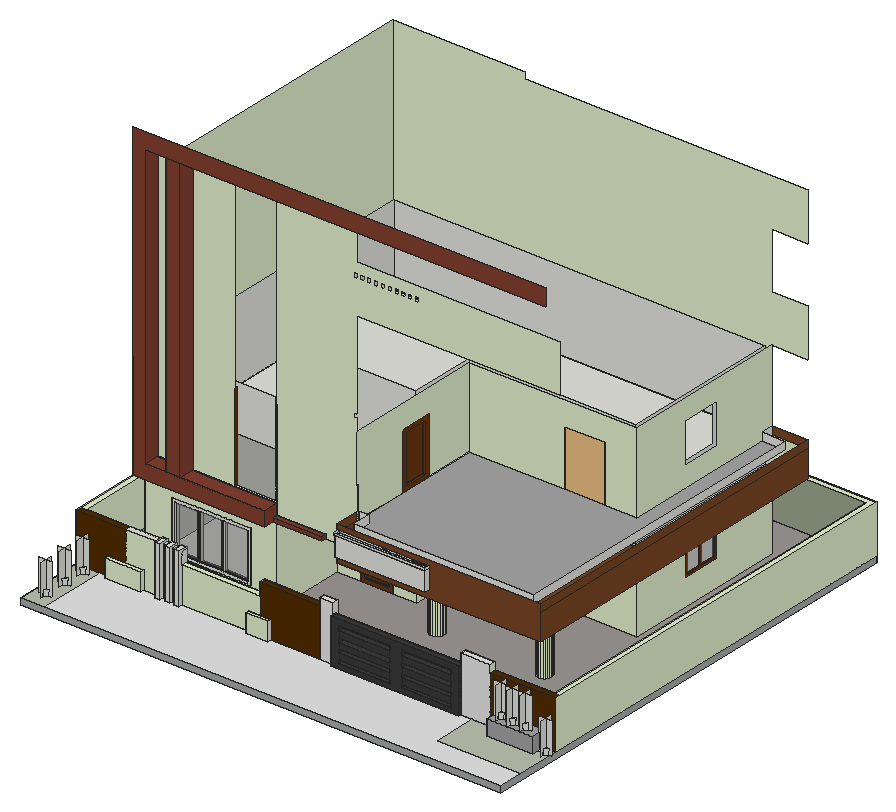
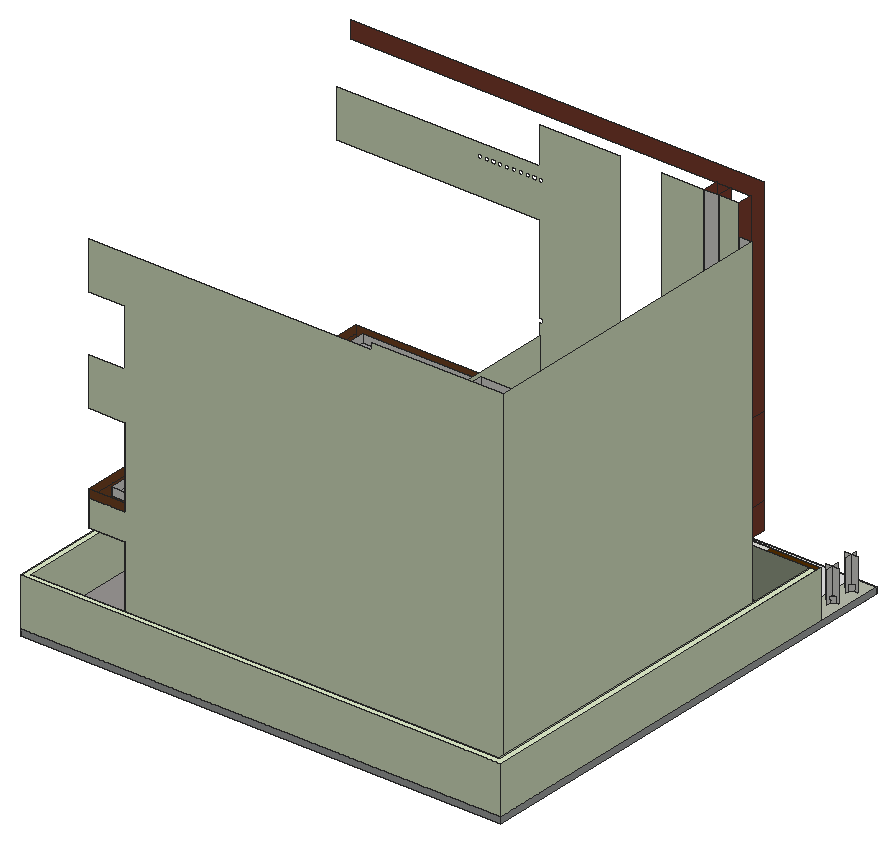
# SketchUp Ruby script. Lengths in inches.
U = 1.inch
M = Sketchup.active_model
def pt(a) = Geom::Point3d.new(a.map { |v| v * U })
def face(e, loops, mat)
  f = e.add_face(loops[0].map { |a| pt(a) })
  loops[1..].each { |l| e.add_face(l.map { |a| pt(a) }).erase! }
  f.material = f.back_material = mat if mat
  f
end
# faces: each face lists its corners as indices into pts; further lists are holes
def faces(e, pts, list, mat = nil) = list.each { |f| face(e, (f[0].is_a?(Array) ? f : [f]).map { |l| l.map { |i| pts[i] } }, mat) }
# xy, xz, yz: faces in a plane at the given z, y or x. An outline is a flat list of corners, or four numbers for a rectangle; further outlines are holes
def ring(l) = l.size == 4 ? [[l[0], l[1]], [l[2], l[1]], [l[2], l[3]], [l[0], l[3]]] : l.each_slice(2).to_a
def flat(e, list, mat, &to3) = list.each { |f| face(e, (f[0].is_a?(Array) ? f : [f]).map { |l| ring(l).map { |u, v| to3.(u, v) } }, mat) }
def xy(e, z, list, mat = nil) = flat(e, list, mat) { |x, y| [x, y, z] }
def xz(e, y, list, mat = nil) = flat(e, list, mat) { |x, z| [x, y, z] }
def yz(e, x, list, mat = nil) = flat(e, list, mat) { |y, z| [x, y, z] }
def lines(e, pts, list) = list.each { |a, b| e.add_line(pt(pts[a]), pt(pts[b])) }
# prism: a flat outline (further loops are holes) pulled along v
def prism(e, loops, v, mat = nil)
  f = face(e, loops, mat); d = Geom::Vector3d.new(v.map { |x| x * U })
  f.pushpull(f.normal.samedirection?(d) ? d.length : -d.length)
end
def box(e, o, s, mat = nil) = prism(e, [[o, [o[0] + s[0], o[1], o[2]], [o[0] + s[0], o[1] + s[1], o[2]], [o[0], o[1] + s[1], o[2]]]], [0, 0, s[2]], mat)
def at(x, y, z, deg = 0) = Geom::Transformation.translation(pt([x, y, z])) * Geom::Transformation.rotation(ORIGIN, Z_AXIS, deg.degrees)
def axes(o, x, y, z) = Geom::Transformation.new([*x, 0, *y, 0, *z, 0, *pt(o).to_a, 1])
def part(name) = M.definitions.add(name)
# library, detail: a bought-in or finely detailed component or shape, given as its bounding box
def library(name, o, s) = part(name).tap { |d| box(d.entities, o, s) }
def detail(e, o, s) = box(e.add_group.entities, o, s)
def put(e, d, t, mat = nil) = e.add_instance(d, t).tap { |i| i.material = mat if mat }
def group(e, t, mat = nil) = e.add_group.tap { |g| g.transformation = t; g.material = mat if mat }.entities
root = M.entities
M.materials.add("[Color A08]").color = [102, 52, 0]
M.materials.add("[Color C08]").color = [82, 45, 0]
M.materials.add("[Color M00]").color = [255, 255, 255]
M.materials.add("[Color M07]").color = [58, 58, 58]
M.materials.add("[Concrete Aggregate Smoke]").color = [154, 150, 148]
M.materials.add("[Concrete Form 4x8]").color = [167, 170, 168]
M.materials.add("[Mirror 01]").color = [185, 185, 181]
M.materials.add("[Pavers Flagstone Gray]").color = [162, 162, 162]
M.materials.add("[Pavers with Grass Brick]").color = [187, 192, 176]
M.materials.add("[Polished Concrete Old]").color = [229, 229, 229]
M.materials.add("[Stone Vein Gray]").color = [166, 165, 165]
M.materials.add("[Translucent Glass Gray]").color = [128, 128, 128]
M.materials["[Translucent Glass Gray]"].alpha = 0.5
M.materials.add("[Wood Board Cork]").color = [130, 63, 47]
M.materials.add("[Wood Lumber ButtJoined]").color = [225, 238, 204]
M.materials.add("[Wood Lumber ButtJoined]1").color = [154, 164, 141]
M.materials.add("[Wood Veneer 01]1").color = [120, 70, 37]
M.materials.add("[Wood Veneer 02]").color = [107, 55, 17]
c1 = part("Gruppe\#59")
xz(c1.entities,0,[[0,0,19.69,47.24]])
c2 = part("Gruppe\#58")
xz(c2.entities,0,[[0,0,19.69,47.24]])
c3 = part("buchsbaum")
xy(c3.entities,8.86,[[9.1875,3.27,15.1,9.1875,9.1875,15.1,3.27,9.1875]])
p = [[9.1875,4.45,0],[9.1875,3.27,8.86],[3.27,9.1875,8.86],[4.45,9.1875,0],[13.92,9.1875,0],[15.1,9.1875,8.86],
  [9.1875,15.1,8.86],[9.1875,13.92,0]]
faces(c3.entities,p,[[0,1,2,3],[4,5,1,0],[3,2,6,7],[7,6,5,4]])
put(c3.entities,c1,at(0,9.84,0))
put(c3.entities,c2,at(9.84,0,0,90))
c4 = part("Group\#3")
xy(c4.entities,0,[[0,0,48,3.1875]],"[Wood Veneer 02]")
xy(c4.entities,5.53,[[5.53,0,42.47,3.1875]],"[Wood Veneer 02]")
xy(c4.entities,78.47,[[5.53,0,42.47,3.1875]],"[Wood Veneer 02]")
xy(c4.entities,84,[[0,0,48,3.1875]],"[Wood Veneer 02]")
xz(c4.entities,0,[[[0,0,48,84],[5.53,5.53,42.47,78.47]]],"[Wood Veneer 02]")
xz(c4.entities,3.1875,[[[0,0,48,84],[5.53,5.53,42.47,78.47]],[5.53,5.53,42.47,78.47]],"[Wood Veneer 02]")
yz(c4.entities,0,[[0,0,3.1875,84]],"[Wood Veneer 02]")
yz(c4.entities,5.53,[[0,5.53,3.1875,78.47]],"[Wood Veneer 02]")
yz(c4.entities,42.47,[[0,5.53,3.1875,78.47]],"[Wood Veneer 02]")
yz(c4.entities,48,[[0,0,3.1875,84]],"[Wood Veneer 02]")
c5 = part("Group\#4")
xy(c5.entities,0,[[0,0,21.9375,1.125]],"[Wood Veneer 02]")
xy(c5.entities,1.52,[[1.52,0,10.45,1.125],[10.97,0,20.42,1.125]],"[Wood Veneer 02]")
xy(c5.entities,22.11,[[1.52,0,10.45,1.125],[10.97,0,20.42,1.125]],"[Wood Veneer 02]")
xy(c5.entities,23.625,[[0,0,21.9375,1.125]],"[Wood Veneer 02]")
xz(c5.entities,0,[[[0,0,21.9375,23.625],[10.97,1.52,20.42,22.11],[1.52,1.52,10.45,22.11]]],"[Wood Veneer 02]")
xz(c5.entities,1.125,[[1.52,1.52,10.45,22.11],[10.97,1.52,20.42,22.11]],"[Translucent Glass Gray]")
xz(c5.entities,1.125,[[[0,0,21.9375,23.625],[10.97,1.52,20.42,22.11],[1.52,1.52,10.45,22.11]]],"[Wood Veneer 02]")
yz(c5.entities,0,[[0,0,1.125,23.625]],"[Wood Veneer 02]")
yz(c5.entities,1.52,[[0,1.52,1.125,22.11]],"[Wood Veneer 02]")
yz(c5.entities,10.45,[[0,1.52,1.125,22.11]],"[Wood Veneer 02]")
yz(c5.entities,10.97,[[0,1.52,1.125,22.11]],"[Wood Veneer 02]")
yz(c5.entities,20.42,[[0,1.52,1.125,22.11]],"[Wood Veneer 02]")
yz(c5.entities,21.9375,[[0,0,1.125,23.625]],"[Wood Veneer 02]")
c6 = part("Group\#2")
xy(c6.entities,0,[[0,0,48,3.1875]],"[Wood Veneer 02]")
xy(c6.entities,5.53,[[5.53,0,42.47,3.1875]],"[Wood Veneer 02]")
xy(c6.entities,78.47,[[5.53,0,42.47,3.1875]],"[Wood Veneer 02]")
xy(c6.entities,84,[[0,0,48,3.1875]],"[Wood Veneer 02]")
xz(c6.entities,0,[[[0,0,48,84],[5.53,5.53,42.47,78.47]]],"[Wood Veneer 02]")
xz(c6.entities,3.1875,[[[0,0,48,84],[5.53,5.53,42.47,78.47]],[5.53,5.53,42.47,78.47]],"[Wood Veneer 02]")
yz(c6.entities,0,[[0,0,3.1875,84]],"[Wood Veneer 02]")
yz(c6.entities,5.53,[[0,5.53,3.1875,78.47]],"[Wood Veneer 02]")
yz(c6.entities,42.47,[[0,5.53,3.1875,78.47]],"[Wood Veneer 02]")
yz(c6.entities,48,[[0,0,3.1875,84]],"[Wood Veneer 02]")
c7 = library("Group\#5",[0,0,0],[60,3.4375,84])
xy(root,0,[[0,0,720,704.375]],"[Concrete Form 4x8]")
xy(root,9,[[47.625,99.125,47.625,104.375,0,104.375,0,704.375,720,704.375,720,104.375,576.98,104.375,576.98,113.375,711,113.375,711,695.375,9,695.375,9,113.375,365.09,113.375,365.09,104.375,101.5,104.375,101.5,99.125],[122.78,99.125,130.4,104.375],[136.78,99.125,144.4,104.375],[150.84,99.125,158.46,104.375],[258.67,99.125,291.92,104.375],
  [53.1875,166.9375,53.1875,631.8125,621.4375,631.8125,621.4375,378.5,543.9375,378.5,543.9375,384.5,615.4375,384.5,615.4375,625.8125,59.1875,625.8125,59.1875,172.9375,245.25,172.9375,245.25,286.0625,286.51,286.0625,286.51,280.0625,251.25,280.0625,251.25,166.9375],[59.1875,172.9375,245.25,172.9375,245.25,286.0625,364.4375,286.0625,364.4375,384.5,615.4375,384.5,615.4375,625.8125,59.1875,625.8125],[431.7,230.58,428.91,230.95,426.32,232.03,424.09,233.73,422.39,235.96,421.3125,238.55,420.95,241.33,421.3125,244.12,422.39,246.71,424.09,248.9375,426.32,250.64,428.91,251.72,431.7,252.08,434.48,251.72,437.07,250.64,439.3,248.9375,441.01,246.71,442.08,244.12,442.45,241.33,442.08,238.55,441.01,235.96,439.3,233.73,437.07,232.03,434.48,230.95],[593.38,230.58,590.6,230.95,588.01,232.03,585.78,233.73,584.07,235.96,583,238.55,582.63,241.33,583,244.12,584.07,246.71,585.78,248.9375,588.01,250.64,590.6,251.72,593.38,252.08,596.17,251.72,598.76,250.64,600.98,248.9375,602.69,246.71,603.77,244.12,604.13,241.33,603.77,238.55,602.69,235.96,600.98,233.73,598.76,232.03,596.17,230.95],[334.51,280.0625,334.51,286.0625,364.4375,286.0625,364.4375,311.76,370.4375,311.76,370.4375,280.0625],
  [364.4375,347.76,364.4375,384.5,495.9375,384.5,495.9375,378.5,370.4375,378.5,370.4375,347.76]])
xy(root,9,[[365.09,104.375,385.78,113.375]],"[Color M00]")
xy(root,9,[[[9,113.375,711,695.375],[53.1875,166.9375,53.1875,631.8125,621.4375,631.8125,621.4375,378.5,543.9375,378.5,543.9375,384.5,495.9375,384.5,495.9375,378.5,370.4375,378.5,370.4375,347.76,364.4375,347.76,364.4375,311.76,370.4375,311.76,370.4375,280.0625,334.51,280.0625,334.51,286.0625,286.51,286.0625,286.51,280.0625,251.25,280.0625,251.25,166.9375],[431.7,230.58,428.91,230.95,426.32,232.03,424.09,233.73,422.39,235.96,421.3125,238.55,420.95,241.33,421.3125,244.12,422.39,246.71,424.09,248.9375,426.32,250.64,428.91,251.72,431.7,252.08,434.48,251.72,437.07,250.64,439.3,248.9375,441.01,246.71,442.08,244.12,442.45,241.33,442.08,238.55,441.01,235.96,439.3,233.73,437.07,232.03,434.48,230.95],[593.38,230.58,590.6,230.95,588.01,232.03,585.78,233.73,584.07,235.96,583,238.55,582.63,241.33,583,244.12,584.07,246.71,585.78,248.9375,588.01,250.64,590.6,251.72,593.38,252.08,596.17,251.72,598.76,250.64,600.98,248.9375,602.69,246.71,603.77,244.12,604.13,241.33,603.77,238.55,602.69,235.96,600.98,233.73,598.76,232.03,596.17,230.95]]],"[Concrete Aggregate Smoke]")
xy(root,9,[[633.14,82.625,701.76,104.375]],"[Pavers Flagstone Gray]")
xy(root,9,[[0,0,35.88,104.375],[593.65,37.8125,720,37.8125,720,104.375,701.76,104.375,701.76,82.625,633.14,82.625,633.14,104.375,593.65,104.375]],"[Pavers with Grass Brick]")
xy(root,9,[[35.88,0,720,0,720,37.8125,593.65,37.8125,593.65,104.375,576.98,104.375,576.98,113.375,385.78,113.375,385.78,104.375,291.92,104.375,291.92,99.125,258.67,99.125,258.67,104.375,158.46,104.375,158.46,99.125,150.84,99.125,150.84,104.375,144.4,104.375,144.4,99.125,136.78,99.125,136.78,104.375,130.4,104.375,130.4,99.125,122.78,99.125,122.78,104.375,101.5,104.375,101.5,99.125,47.625,99.125,47.625,104.375,35.88,104.375]],"[Polished Concrete Old]")
xy(root,26.23,[[93.41,166.9375,212.47,172.9375]])
xy(root,33,[[633.14,82.625,701.76,104.375]],"[Pavers Flagstone Gray]")
xy(root,36.4375,[[47.625,99.125,101.5,104.375],[258.67,99.125,291.92,104.375]],"[Wood Lumber ButtJoined]")
xy(root,41.18,[[404.68,378.5,470.49,384.5]])
xy(root,47.24,[[615.4375,469.14,621.4375,529.14]])
xy(root,62.8125,[[158.46,104.375,275.3,113.375]],"[Wood Lumber ButtJoined]")
xy(root,81,[[74.5625,104.375,122.78,113.375],[122.78,104.375,130.4,113.375],[136.78,104.375,144.4,113.375],[150.84,104.375,158.46,113.375]])
xy(root,81,[[0,104.375,74.5625,113.375],[275.3,104.375,365.09,113.375],[621.03,104.375,720,113.375]],"[Color C08]")
xy(root,81,[[130.4,104.375,136.78,113.375],[144.4,104.375,150.84,113.375],[0,113.375,9,113.375,9,695.375,711,695.375,711,113.375,720,113.375,720,704.375,0,704.375]],"[Wood Lumber ButtJoined]")
xy(root,83.5625,[[122.78,99.125,130.4,113.375],[136.78,99.125,144.4,113.375],[150.84,99.125,158.46,113.375]])
xy(root,91.5625,[[365.09,104.375,385.78,113.375],[576.98,104.375,621.03,113.375]],"[Polished Concrete Old]")
xy(root,93,[[286.51,280.0625,334.51,286.0625],[364.4375,311.76,370.4375,347.76],[495.9375,378.5,543.9375,384.5]])
xy(root,96.3,[[404.68,378.5,470.49,384.5]])
xy(root,103.79,[[93.41,166.9375,212.47,172.9375]])
xy(root,107.24,[[615.4375,469.14,621.4375,529.14]])
xy(root,129,[[431.7,230.58,434.48,230.95,437.07,232.03,439.3,233.73,441.01,235.96,442.08,238.55,442.45,241.33,442.08,244.12,441.01,246.71,439.3,248.9375,437.07,250.64,434.48,251.72,431.7,252.08,428.91,251.72,426.32,250.64,424.09,248.9375,422.39,246.71,421.3125,244.12,420.95,241.33,421.3125,238.55,422.39,235.96,424.09,233.73,426.32,232.03,428.91,230.95],[593.38,230.58,596.17,230.95,598.76,232.03,600.98,233.73,602.69,235.96,603.77,238.55,604.13,241.33,603.77,244.12,602.69,246.71,600.98,248.9375,598.76,250.64,596.17,251.72,593.38,252.08,590.6,251.72,588.01,250.64,585.78,248.9375,584.07,246.71,583,244.12,582.63,241.33,583,238.55,584.07,235.96,585.78,233.73,588.01,232.03,590.6,230.95]])
xy(root,129,[[53.1875,144.0625,53.1875,166.9375,324.3125,166.9375,324.3125,159,251.25,159,251.25,144.0625]],"[Wood Board Cork]")
xy(root,129,[[251.25,166.9375,370.4375,280.0625]],"[Wood Lumber ButtJoined]1")
xy(root,129,[[370.4375,131.0625,675.3125,378.5],[621.4375,378.5,675.3125,631.8125]],"[Wood Veneer 01]1")
xy(root,134.97,[[251.25,159,324.3125,166.9375]],"[Wood Board Cork]")
xy(root,140.85,[[373.11,123.75,506.92,131.0625]])
xy(root,151.14,[[103.04,144.0625,124.63,166.9375],[187.94,166.9375,251.25,171.5625]])
xy(root,151.14,[[72.33,144.0625,103.04,166.9375],[124.63,144.0625,251.25,166.9375]],"[Wood Board Cork]")
xy(root,165.1875,[[59.1875,172.9375,59.1875,625.8125,615.4375,625.8125,615.4375,384.5,364.4375,384.5,364.4375,286.0625,245.25,286.0625,245.25,172.9375]])
xy(root,169.0625,[[59.1875,172.9375,245.25,172.9375,245.25,286.0625,364.4375,286.0625,364.4375,384.5,615.4375,384.5,615.4375,625.8125,59.1875,625.8125],[364.4375,253.7,370.4375,280.0625],[364.4375,280.0625,370.4375,301.7]])
xy(root,169.0625,[[385.875,142.1875,656.91,142.1875,656.91,612.27,621.4375,612.27,621.4375,378.5,572.99,378.5,572.99,384.5,512.99,384.5,512.99,378.5,370.4375,378.5,370.4375,170.75,385.875,170.75]],"[Stone Vein Gray]")
xy(root,170.48,[[371.79,122.6875,508.29,123.75],[371.79,123.75,373.11,131.0625],[373.11,123.75,506.92,131.0625],[506.92,123.75,508.29,131.0625]])
xz(root,0,[[0,0,720,9]],"[Concrete Form 4x8]")
xz(root,82.625,[[633.14,9,701.76,33]],"[Pavers Flagstone Gray]")
xz(root,99.125,[[122.78,9,130.4,83.5625],[136.78,9,144.4,83.5625],[150.84,9,158.46,83.5625]])
xz(root,99.125,[[47.625,9,101.5,36.4375],[258.67,9,291.92,36.4375]],"[Wood Lumber ButtJoined]")
xz(root,104.375,[[122.78,9,130.4,81],[136.78,9,144.4,81],[150.84,9,158.46,81],[258.67,9,291.92,36.4375]])
xz(root,104.375,[[0,9,47.625,9,47.625,36.4375,74.5625,36.4375,74.5625,81,0,81],[291.92,9,365.09,9,365.09,81,275.3,81,275.3,36.4375,291.92,36.4375],[621.03,9,633.14,9,633.14,33,701.76,33,701.76,9,720,9,720,81,621.03,81]],"[Color C08]")
xz(root,104.375,[[633.14,9,701.76,33]],"[Pavers Flagstone Gray]")
xz(root,104.375,[[365.09,9,385.78,91.5625],[576.98,9,621.03,91.5625]],"[Polished Concrete Old]")
xz(root,104.375,[[101.5,9,122.78,9,122.78,81,74.5625,81,74.5625,36.4375,101.5,36.4375],[130.4,9,136.78,81],[144.4,9,150.84,81],[158.46,9,258.67,9,258.67,36.4375,275.3,36.4375,275.3,62.8125,158.46,62.8125]],"[Wood Lumber ButtJoined]")
xz(root,113.375,[[122.78,81,130.4,83.5625],[136.78,81,144.4,83.5625],[150.84,81,158.46,83.5625]])
xz(root,113.375,[[365.09,9,385.78,91.5625]],"[Polished Concrete Old]")
xz(root,113.375,[[9,9,9,81,158.46,81,158.46,62.8125,275.3,62.8125,275.3,81,365.09,81,365.09,9],[576.98,9,576.98,91.5625,621.03,91.5625,621.03,81,711,81,711,9]],"[Wood Lumber ButtJoined]1")
xz(root,122.6875,[[371.79,170.48,508.29,173.23]])
xz(root,123.75,[[373.11,140.85,506.92,170.48]])
xz(root,131.0625,[[373.11,140.85,506.92,170.48],[371.79,170.48,508.29,173.23]])
xz(root,131.0625,[[[370.4375,129,675.3125,181.0625],[373.11,140.85,373.11,170.48,371.79,170.48,371.79,173.23,508.29,173.23,508.29,170.48,506.92,170.48,506.92,140.85]]],"[Wood Veneer 01]1")
xz(root,142.1875,[[385.875,169.0625,656.91,181.0625]])
xz(root,144.0625,[[53.1875,129,251.25,129,251.25,151.14,72.33,151.14,72.33,572.45,672.375,572.45,672.375,597.6875,53.1875,597.6875],[103.04,151.14,124.63,572.45]],"[Wood Board Cork]")
xz(root,159,[[251.25,129,324.3125,134.97]],"[Wood Board Cork]")
xz(root,166.9375,[[53.1875,129,53.1875,526.5,72.33,526.5,72.33,151.14,251.25,151.14,251.25,129],[103.04,151.14,124.63,572.45]])
xz(root,166.9375,[[251.25,129,324.3125,134.97]],"[Wood Board Cork]")
xz(root,166.9375,[[[53.1875,9,251.25,129],[93.41,26.23,212.47,103.79]],[[324.3125,129,370.4375,129,370.4375,307.4375,365.79,307.4375,365.79,313.15,370.4375,313.15,370.4375,445.0625,675.875,445.0625,675.875,517.0625,370.4375,517.0625,370.4375,572.45,251.25,572.45,251.25,134.97,324.3125,134.97],[458.04,495.42,464.47,501.86],[447.79,495.42,454.22,501.86],[437.54,495.42,443.97,501.86],[427.29,495.42,433.72,501.86],[417.04,495.42,423.47,501.86],[406.79,495.42,413.22,501.86],[396.54,495.42,402.97,501.86],[386.29,495.42,392.72,501.86],[376.04,495.42,382.47,501.86],[365.79,495.42,372.22,501.86]],[72.33,151.14,103.04,572.45],[124.63,151.14,187.94,572.45]],"[Wood Lumber ButtJoined]")
xz(root,170.75,[[370.4375,169.0625,385.875,181.0625]])
xz(root,171.5625,[[187.94,151.14,251.25,219.24]],"[Mirror 01]")
xz(root,172.9375,[[[59.1875,9,245.25,129],[93.41,26.23,212.47,103.79]],[59.1875,129,245.25,165.1875],[59.1875,165.1875,245.25,169.0625],[59.1875,169.0625,245.25,289.0625]])
xz(root,253.7,[[364.4375,169.0625,370.4375,253.0625]])
xz(root,280.0625,[[251.25,129,370.4375,169.0625]])
xz(root,280.0625,[[251.25,9,286.51,9,286.51,93,334.51,93,334.51,9,370.4375,9,370.4375,129,251.25,129]],"[Wood Lumber ButtJoined]")
xz(root,286.0625,[[245.25,9,245.25,129,364.4375,129,364.4375,9,334.51,9,334.51,93,286.51,93,286.51,9],[245.25,129,364.4375,165.1875],[245.25,165.1875,304.84,169.0625],[304.84,165.1875,326.48,169.0625],[326.48,165.1875,364.4375,169.0625],
  [245.25,169.0625,364.4375,289.0625]])
xz(root,301.7,[[364.4375,169.0625,370.4375,253.0625]])
xz(root,311.76,[[364.4375,9,370.4375,93]])
xz(root,347.76,[[364.4375,9,370.4375,93]])
xz(root,378.5,[[[370.4375,9,495.9375,9,495.9375,93,543.9375,93,543.9375,9,621.4375,9,621.4375,129,370.4375,129],[404.68,41.18,470.49,96.3]],[370.4375,169.0625,512.99,169.0625,512.99,253.0625,572.99,253.0625,572.99,169.0625,621.4375,169.0625,621.4375,289.0625,370.4375,289.0625]],"[Wood Lumber ButtJoined]")
xz(root,384.5,[[[364.4375,9,364.4375,129,615.4375,129,615.4375,9,543.9375,9,543.9375,93,495.9375,93,495.9375,9],[404.68,41.18,470.49,96.3]],[364.4375,129,615.4375,165.1875],[364.4375,165.1875,615.4375,169.0625],[364.4375,169.0625,364.4375,289.0625,615.4375,289.0625,615.4375,169.0625,572.99,169.0625,572.99,253.0625,512.99,253.0625,512.99,169.0625]])
xz(root,469.14,[[615.4375,47.24,621.4375,107.24]])
xz(root,529.14,[[615.4375,47.24,621.4375,107.24]])
xz(root,612.27,[[621.4375,169.0625,656.91,181.0625]])
xz(root,625.8125,[[59.1875,9,615.4375,165.1875],[59.1875,165.1875,615.4375,169.0625],[59.1875,169.0625,615.4375,289.0625]])
xz(root,631.8125,[[53.1875,9,53.1875,526.5,251.25,526.5,251.25,517.0625,675.875,517.0625,675.875,445.0625,621.4375,445.0625,621.4375,361.0625,675.875,361.0625,675.875,289.0625,621.4375,289.0625,621.4375,169.0625,675.3125,169.0625,675.3125,129,621.4375,129,621.4375,9]],"[Wood Lumber ButtJoined]")
xz(root,631.8125,[[621.4375,169.0625,675.3125,181.0625]],"[Wood Veneer 01]1")
xz(root,695.375,[[9,9,711,81]],"[Wood Lumber ButtJoined]1")
xz(root,704.375,[[0,0,720,9]],"[Concrete Form 4x8]")
xz(root,704.375,[[0,9,720,81]],"[Wood Lumber ButtJoined]")
yz(root,0,[[0,0,704.375,9]],"[Concrete Form 4x8]")
yz(root,0,[[104.375,9,704.375,81]],"[Wood Lumber ButtJoined]")
yz(root,9,[[113.375,9,695.375,81]],"[Wood Lumber ButtJoined]")
yz(root,47.625,[[99.125,9,104.375,36.4375]],"[Wood Lumber ButtJoined]")
yz(root,53.1875,[[144.0625,129,166.9375,169.0625],[144.0625,169.0625,166.9375,289.0625]],"[Wood Board Cork]")
yz(root,53.1875,[[166.9375,9,631.8125,526.5]],"[Wood Lumber ButtJoined]")
yz(root,59.1875,[[172.9375,9,625.8125,129],[172.9375,129,625.8125,165.1875],[172.9375,165.1875,625.8125,169.0625],[172.9375,169.0625,625.8125,289.0625]])
yz(root,72.33,[[144.0625,151.14,166.9375,572.45]],"[Wood Board Cork]")
yz(root,93.41,[[166.9375,26.23,172.9375,103.79]])
yz(root,101.5,[[99.125,9,104.375,36.4375]],"[Wood Lumber ButtJoined]")
yz(root,103.04,[[144.0625,151.14,166.9375,572.45]],"[Wood Board Cork]")
yz(root,122.78,[[99.125,9,99.125,83.5625,113.375,83.5625,113.375,81,104.375,81,104.375,9]])
yz(root,124.63,[[144.0625,151.14,166.9375,572.45]],"[Wood Board Cork]")
yz(root,130.4,[[99.125,9,104.375,9,104.375,81,113.375,81,113.375,83.5625,99.125,83.5625]])
yz(root,136.78,[[99.125,9,99.125,83.5625,113.375,83.5625,113.375,81,104.375,81,104.375,9]])
yz(root,144.4,[[99.125,9,104.375,9,104.375,81,113.375,81,113.375,83.5625,99.125,83.5625]])
yz(root,150.84,[[99.125,9,99.125,83.5625,113.375,83.5625,113.375,81,104.375,81,104.375,9]])
yz(root,158.46,[[99.125,9,104.375,9,104.375,81,113.375,81,113.375,83.5625,99.125,83.5625],[104.375,62.8125,113.375,81]])
yz(root,187.94,[[166.9375,151.14,171.5625,282.65]],"[Color A08]")
yz(root,212.47,[[166.9375,26.23,172.9375,103.79]])
yz(root,245.25,[[172.9375,9,286.0625,129],[172.9375,129,286.0625,165.1875],[172.9375,165.1875,286.0625,169.0625],[172.9375,169.0625,286.0625,289.0625]])
yz(root,251.25,[[166.9375,129,280.0625,129,280.0625,169.0625,171.5625,169.0625,171.5625,151.14,166.9375,151.14]])
yz(root,251.25,[[166.9375,151.14,171.5625,169.0625],[166.9375,169.0625,171.5625,282.65]],"[Color A08]")
yz(root,251.25,[[144.0625,129,159,129,159,134.97,166.9375,134.97,166.9375,151.14,144.0625,151.14]],"[Wood Board Cork]")
yz(root,251.25,[[166.9375,9,280.0625,129]],"[Wood Lumber ButtJoined]")
yz(root,258.67,[[99.125,9,104.375,36.4375]])
yz(root,275.3,[[104.375,62.8125,113.375,81]])
yz(root,286.51,[[280.0625,9,286.0625,93]])
yz(root,291.92,[[99.125,9,104.375,36.4375]])
yz(root,324.3125,[[159,129,166.9375,134.97]],"[Wood Board Cork]")
yz(root,334.51,[[280.0625,9,286.0625,93]])
yz(root,364.4375,[[286.0625,9,286.0625,129,384.5,129,384.5,9,347.76,9,347.76,93,311.76,93,311.76,9],[286.0625,129,384.5,165.1875],[286.0625,165.1875,384.5,169.0625],[253.7,169.0625,286.0625,253.0625],[286.0625,169.0625,301.7,253.0625],
  [301.7,169.0625,301.7,253.0625,286.0625,253.0625,286.0625,289.0625,384.5,289.0625,384.5,169.0625]])
yz(root,365.09,[[104.375,9,113.375,81]],"[Color M00]")
yz(root,365.09,[[104.375,81,113.375,91.5625]],"[Polished Concrete Old]")
yz(root,370.4375,[[166.9375,129,280.0625,169.0625],[280.0625,129,378.5,169.0625],[166.9375,169.0625,170.75,181.0625]])
yz(root,370.4375,[[280.0625,9,311.76,9,311.76,93,347.76,93,347.76,9,378.5,9,378.5,129,280.0625,129],[170.75,169.0625,253.7,169.0625,253.7,253.0625,301.7,253.0625,301.7,169.0625,378.5,169.0625,378.5,289.0625,166.9375,289.0625,166.9375,217.0625,170.75,217.0625]],"[Wood Lumber ButtJoined]")
yz(root,370.4375,[[131.0625,129,166.9375,169.0625],[131.0625,169.0625,166.9375,181.0625]],"[Wood Veneer 01]1")
yz(root,371.79,[[122.6875,170.48,131.0625,173.23]])
yz(root,373.11,[[123.75,140.85,131.0625,170.48]])
yz(root,385.78,[[104.375,9,113.375,91.5625]],"[Polished Concrete Old]")
yz(root,385.875,[[142.1875,169.0625,170.75,181.0625]])
yz(root,404.68,[[378.5,41.18,384.5,96.3]])
yz(root,470.49,[[378.5,41.18,384.5,96.3]])
yz(root,495.9375,[[378.5,9,384.5,93]])
yz(root,506.92,[[123.75,140.85,131.0625,170.48]])
yz(root,508.29,[[122.6875,170.48,131.0625,173.23]])
yz(root,512.99,[[378.5,169.0625,384.5,253.0625]])
yz(root,543.9375,[[378.5,9,384.5,93]])
yz(root,572.99,[[378.5,169.0625,384.5,253.0625]])
yz(root,576.98,[[104.375,9,113.375,91.5625]],"[Polished Concrete Old]")
yz(root,615.4375,[[[384.5,9,625.8125,129],[469.14,47.24,529.14,107.24]],[384.5,129,625.8125,165.1875],[384.5,165.1875,625.8125,169.0625],[[384.5,169.0625,625.8125,289.0625],[469.14,198.99,529.14,258.99]]])
yz(root,621.03,[[104.375,81,113.375,91.5625]],"[Wood Lumber ButtJoined]")
yz(root,621.4375,[[612.27,169.0625,631.8125,169.0625,631.8125,181.0625,624.5625,181.0625,624.5625,217.0625,622.04,217.0625,622.04,181.0625,612.27,181.0625]])
yz(root,621.4375,[[[378.5,9,631.8125,129],[469.14,47.24,529.14,107.24]],[[378.5,169.0625,612.27,169.0625,612.27,181.0625,622.04,181.0625,622.04,218.3125,624.5625,218.3125,624.5625,181.0625,631.8125,181.0625,631.8125,289.0625,378.5,289.0625],[469.14,198.99,529.14,258.99]]],"[Wood Lumber ButtJoined]")
yz(root,633.14,[[82.625,9,104.375,33]],"[Pavers Flagstone Gray]")
yz(root,656.91,[[142.1875,169.0625,612.27,181.0625]])
yz(root,675.3125,[[131.0625,129,631.8125,169.0625],[131.0625,169.0625,631.8125,181.0625]],"[Wood Veneer 01]1")
yz(root,701.76,[[82.625,9,104.375,33]],"[Pavers Flagstone Gray]")
yz(root,711,[[113.375,9,695.375,81]],"[Wood Lumber ButtJoined]")
yz(root,720,[[0,0,704.375,9]],"[Concrete Form 4x8]")
yz(root,720,[[104.375,9,704.375,81]],"[Wood Lumber ButtJoined]")
p = [[428.91,230.95,9],[431.7,230.58,9],[431.7,230.58,129],[428.91,230.95,129],[434.48,230.95,9],[434.48,230.95,129],
  [590.6,230.95,9],[593.38,230.58,9],[593.38,230.58,129],[590.6,230.95,129],[596.17,230.95,9],[596.17,230.95,129],
  [426.32,232.03,9],[426.32,232.03,129],[437.07,232.03,9],[437.07,232.03,129],[588.01,232.03,9],[588.01,232.03,129],
  [598.76,232.03,9],[598.76,232.03,129],[424.09,233.73,9],[424.09,233.73,129],[439.3,233.73,9],[439.3,233.73,129],
  [585.78,233.73,9],[585.78,233.73,129],[600.98,233.73,9],[600.98,233.73,129],[422.39,235.96,9],[422.39,235.96,129],
  [441.01,235.96,9],[441.01,235.96,129],[584.07,235.96,9],[584.07,235.96,129],[602.69,235.96,9],[602.69,235.96,129],
  [421.3125,238.55,9],[421.3125,238.55,129],[442.08,238.55,9],[442.08,238.55,129],[583,238.55,9],[583,238.55,129],
  [603.77,238.55,9],[603.77,238.55,129],[420.95,241.33,9],[420.95,241.33,129],[442.45,241.33,9],[442.45,241.33,129],
  [582.63,241.33,9],[582.63,241.33,129],[604.13,241.33,9],[604.13,241.33,129],[421.3125,244.12,9],[421.3125,244.12,129],
  [442.08,244.12,9],[442.08,244.12,129],[583,244.12,9],[583,244.12,129],[603.77,244.12,9],[603.77,244.12,129],
  [422.39,246.71,9],[422.39,246.71,129],[441.01,246.71,9],[441.01,246.71,129],[584.07,246.71,9],[584.07,246.71,129],
  [602.69,246.71,9],[602.69,246.71,129],[424.09,248.9375,9],[424.09,248.9375,129],[439.3,248.9375,9],[439.3,248.9375,129],
  [585.78,248.9375,9],[585.78,248.9375,129],[600.98,248.9375,9],[600.98,248.9375,129],[426.32,250.64,9],[426.32,250.64,129],
  [437.07,250.64,9],[437.07,250.64,129],[588.01,250.64,9],[588.01,250.64,129],[598.76,250.64,9],[598.76,250.64,129],
  [428.91,251.72,9],[428.91,251.72,129],[434.48,251.72,9],[434.48,251.72,129],[590.6,251.72,9],[590.6,251.72,129],
  [596.17,251.72,9],[596.17,251.72,129],[431.7,252.08,9],[431.7,252.08,129],[593.38,252.08,9],[593.38,252.08,129],
  [187.94,166.9375,151.14],[187.94,166.9375,139.52]]
faces(root,p,[[0,1,2,3],[1,4,5,2],[6,7,8,9],[7,10,11,8],[12,0,3,13],[4,14,15,5],[16,6,9,17],[10,18,19,11],
  [20,12,13,21],[14,22,23,15],[24,16,17,25],[18,26,27,19],[28,20,21,29],[22,30,31,23],[32,24,25,33],[26,34,35,27],
  [36,28,29,37],[30,38,39,31],[40,32,33,41],[34,42,43,35],[44,36,37,45],[38,46,47,39],[48,40,41,49],[42,50,51,43],
  [52,44,45,53],[46,54,55,47],[56,48,49,57],[50,58,59,51],[60,52,53,61],[54,62,63,55],[64,56,57,65],[58,66,67,59],
  [68,60,61,69],[62,70,71,63],[72,64,65,73],[66,74,75,67],[76,68,69,77],[70,78,79,71],[80,72,73,81],[74,82,83,75],
  [84,76,77,85],[78,86,87,79],[88,80,81,89],[82,90,91,83],[92,84,85,93],[86,92,93,87],[94,88,89,95],[90,94,95,91]],"[Wood Lumber ButtJoined]")
lines(root,p,[[96,97]])
put(root,c3,at(8.85,83.03,9))
put(root,c3,at(8.85,49.4,9))
put(root,c3,at(8.85,14.34,9))
put(root,c4,axes([369.45,311.93,9],[0,0.7465,0],[-0.6912,0,0],[0,0,1.00224]))
g1 = group(root,at(385.78,99.86,9))
xy(g1,0,[[0,0,191.2,9.67]],"[Color M07]")
xy(g1,7.52,[[11.42,0,87.68,9.67],[106.08,0,179.78,9.67]],"[Color M07]")
xy(g1,12.37,[[11.42,0,87.68,9.67],[106.08,0,179.78,9.67]],"[Color M07]")
xy(g1,21.13,[[11.42,0,87.68,9.67],[106.08,0,179.78,9.67]],"[Color M07]")
xy(g1,26.8,[[11.42,0,87.68,9.67],[106.08,0,179.78,9.67]],"[Color M07]")
xy(g1,35.5625,[[11.42,0,87.68,9.67],[106.08,0,179.78,9.67]],"[Color M07]")
xy(g1,41.97,[[11.42,0,87.68,9.67],[106.08,0,179.78,9.67]],"[Color M07]")
xy(g1,50.73,[[11.42,0,87.68,9.67],[106.08,0,179.78,9.67]],"[Color M07]")
xy(g1,59.34,[[11.42,0,87.68,9.67],[106.08,0,179.78,9.67]],"[Color M07]")
xy(g1,66.86,[[0,0,191.2,9.67]],"[Color M07]")
xz(g1,0,[[[0,0,191.2,66.86],[11.42,7.52,87.68,59.34],[106.08,7.52,179.78,59.34]],[11.42,12.37,87.68,21.13],[106.08,12.37,179.78,21.13],[11.42,26.8,87.68,35.5625],[106.08,26.8,179.78,35.5625],
  [11.42,41.97,87.68,50.73],[106.08,41.97,179.78,50.73]],"[Color M07]")
xz(g1,9.67,[[[0,0,191.2,66.86],[11.42,50.73,87.68,59.34],[106.08,50.73,179.78,59.34],[11.42,35.5625,87.68,41.97],[106.08,35.5625,179.78,41.97],[11.42,21.13,87.68,26.8],[106.08,21.13,179.78,26.8],[11.42,7.52,87.68,12.37],[106.08,7.52,179.78,12.37]]],"[Color M07]")
yz(g1,0,[[0,0,9.67,66.86]],"[Color M07]")
yz(g1,11.42,[[0,7.52,9.67,12.37],[0,21.13,9.67,26.8],[0,35.5625,9.67,41.97],[0,50.73,9.67,59.34]],"[Color M07]")
yz(g1,87.68,[[0,7.52,9.67,12.37],[0,21.13,9.67,26.8],[0,35.5625,9.67,41.97],[0,50.73,9.67,59.34]],"[Color M07]")
yz(g1,106.08,[[0,7.52,9.67,12.37],[0,21.13,9.67,26.8],[0,35.5625,9.67,41.97],[0,50.73,9.67,59.34]],"[Color M07]")
yz(g1,179.78,[[0,7.52,9.67,12.37],[0,21.13,9.67,26.8],[0,35.5625,9.67,41.97],[0,50.73,9.67,59.34]],"[Color M07]")
yz(g1,191.2,[[0,0,9.67,66.86]],"[Color M07]")
put(root,c3,at(702.71,84.1875,9))
put(root,c4,at(495.9375,378.5,9))
put(root,c4,at(286.51,280.0625,9))
g2 = group(root,at(93.41,166.9375,26.23))
xy(g2,0,[[0,0,119.0625,6.1875]])
xy(g2,4.41,[[5.02,0,38.6,2.8125],[41.67,0,74.78,2.8125],[77.86,0,114.04,2.8125],[5.02,2.8125,38.6,6.1875],[41.67,2.8125,74.78,6.1875],
  [77.86,2.8125,114.04,6.1875]])
xy(g2,73.15,[[5.02,0,38.6,2.8125],[41.67,0,74.78,2.8125],[77.86,0,114.04,2.8125],[5.02,2.8125,38.6,6.1875],[41.67,2.8125,74.78,6.1875],
  [77.86,2.8125,114.04,6.1875]])
xy(g2,77.5625,[[0,0,119.0625,6.1875]])
xz(g2,0,[[[0,0,119.0625,77.5625],[77.86,4.41,114.04,73.15],[5.02,4.41,38.6,73.15],[41.67,4.41,74.78,73.15]]])
xz(g2,2.8125,[[5.02,4.41,38.6,73.15],[41.67,4.41,74.78,73.15],[77.86,4.41,114.04,73.15]],"[Translucent Glass Gray]")
xz(g2,6.1875,[[[0,0,119.0625,77.5625],[77.86,4.41,114.04,73.15],[5.02,4.41,38.6,73.15],[41.67,4.41,74.78,73.15]]])
yz(g2,0,[[0,0,6.1875,77.5625]])
yz(g2,5.02,[[0,4.41,2.8125,73.15],[2.8125,4.41,6.1875,73.15]])
yz(g2,38.6,[[0,4.41,2.8125,73.15],[2.8125,4.41,6.1875,73.15]])
yz(g2,41.67,[[0,4.41,2.8125,73.15],[2.8125,4.41,6.1875,73.15]])
yz(g2,74.78,[[0,4.41,2.8125,73.15],[2.8125,4.41,6.1875,73.15]])
yz(g2,77.86,[[0,4.41,2.8125,73.15],[2.8125,4.41,6.1875,73.15]])
yz(g2,114.04,[[0,4.41,2.8125,73.15],[2.8125,4.41,6.1875,73.15]])
yz(g2,119.0625,[[0,0,6.1875,77.5625]])
put(root,c3,at(634.91,84.6,33))
put(root,c3,at(653.82,82.625,33))
put(root,c3,at(673.01,82.625,33))
put(root,c5,axes([404.68,378.5,41.18],[3,0,0],[0,2,0],[0,0,2.33333]))
put(root,c5,axes([621.26,468.59,47.24],[0,2.76,0],[-1.84,0,0],[0,0,2.53968]))
put(root,c6,axes([370.4375,254.04,169.0625],[0,0.99284,0],[-1.31328,0,0],[0,0,1.00224]))
put(root,c7,at(512.99,378.5,169.0625))
